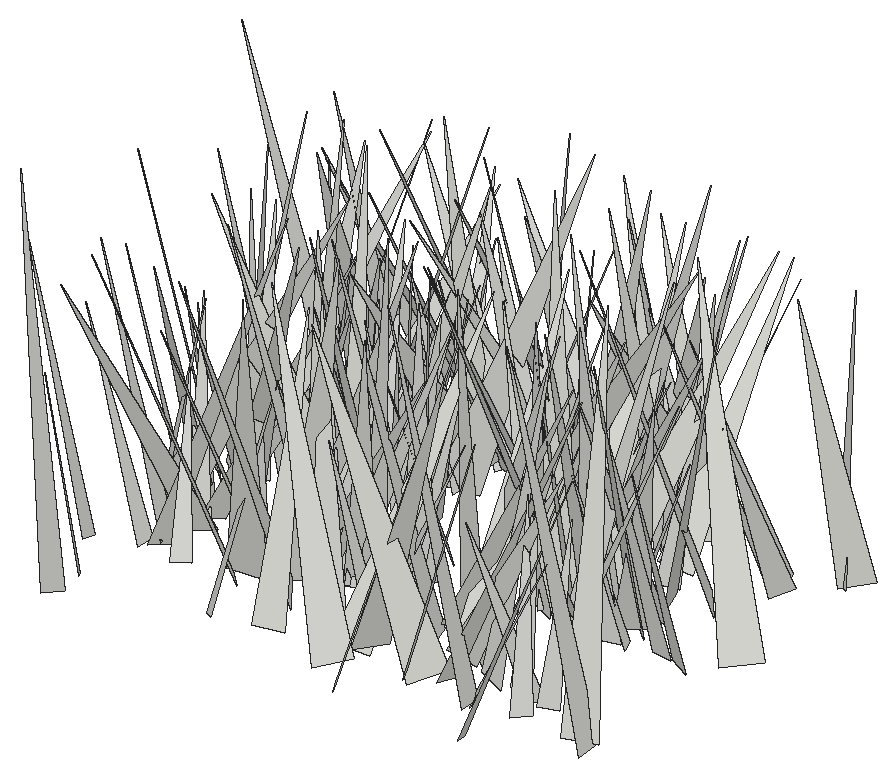
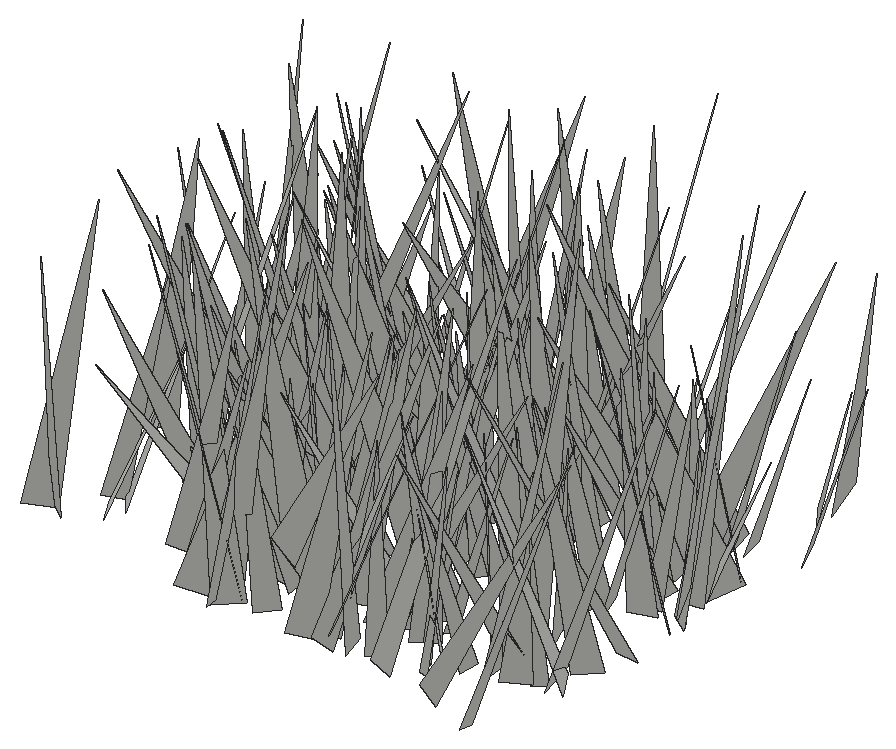
# SketchUp Ruby script. Lengths in inches.
U = 1.inch
M = Sketchup.active_model
def pt(a) = Geom::Point3d.new(a.map { |v| v * U })
def face(e, loops, mat)
  f = e.add_face(loops[0].map { |a| pt(a) })
  loops[1..].each { |l| e.add_face(l.map { |a| pt(a) }).erase! }
  f.material = f.back_material = mat if mat
  f
end
# faces: each face lists its corners as indices into pts; further lists are holes
def faces(e, pts, list, mat = nil) = list.each { |f| face(e, (f[0].is_a?(Array) ? f : [f]).map { |l| l.map { |i| pts[i] } }, mat) }
# xy, xz, yz: faces in a plane at the given z, y or x. An outline is a flat list of corners, or four numbers for a rectangle; further outlines are holes
def ring(l) = l.size == 4 ? [[l[0], l[1]], [l[2], l[1]], [l[2], l[3]], [l[0], l[3]]] : l.each_slice(2).to_a
def flat(e, list, mat, &to3) = list.each { |f| face(e, (f[0].is_a?(Array) ? f : [f]).map { |l| ring(l).map { |u, v| to3.(u, v) } }, mat) }
def xy(e, z, list, mat = nil) = flat(e, list, mat) { |x, y| [x, y, z] }
def xz(e, y, list, mat = nil) = flat(e, list, mat) { |x, z| [x, y, z] }
def yz(e, x, list, mat = nil) = flat(e, list, mat) { |y, z| [x, y, z] }
def lines(e, pts, list) = list.each { |a, b| e.add_line(pt(pts[a]), pt(pts[b])) }
# prism: a flat outline (further loops are holes) pulled along v
def prism(e, loops, v, mat = nil)
  f = face(e, loops, mat); d = Geom::Vector3d.new(v.map { |x| x * U })
  f.pushpull(f.normal.samedirection?(d) ? d.length : -d.length)
end
def box(e, o, s, mat = nil) = prism(e, [[o, [o[0] + s[0], o[1], o[2]], [o[0] + s[0], o[1] + s[1], o[2]], [o[0], o[1] + s[1], o[2]]]], [0, 0, s[2]], mat)
def at(x, y, z, deg = 0) = Geom::Transformation.translation(pt([x, y, z])) * Geom::Transformation.rotation(ORIGIN, Z_AXIS, deg.degrees)
def axes(o, x, y, z) = Geom::Transformation.new([*x, 0, *y, 0, *z, 0, *pt(o).to_a, 1])
def part(name) = M.definitions.add(name)
# library, detail: a bought-in or finely detailed component or shape, given as its bounding box
def library(name, o, s) = part(name).tap { |d| box(d.entities, o, s) }
def detail(e, o, s) = box(e.add_group.entities, o, s)
def put(e, d, t, mat = nil) = e.add_instance(d, t).tap { |i| i.material = mat if mat }
def group(e, t, mat = nil) = e.add_group.tap { |g| g.transformation = t; g.material = mat if mat }.entities
root = M.entities
c1 = part("fur_instance\#9")
p = [[0.8125,0,1.79],[0.67,-0.02,1.48],[0,-0.11,0],[0,0.11,0]]
faces(c1.entities,p,[[0,1,2,3]])
put(root,c1,axes([66.11,216.6875,-27.1],[-3.1769,-1.92196,0.83625],[-2.09296,2.82701,-1.45378],[-0.11299,1.67333,3.4166]))
put(root,c1,axes([66.16,215.04,-27.1],[-7.80069,-0.47128,0.71432],[-0.70737,7.23754,-2.94972],[0.48165,2.99651,7.23686]))
put(root,c1,axes([73.01,220.41,-27.1],[-6.10663,-5.12788,1.30944],[-4.81653,6.21333,1.86984],[2.19336,-0.63253,7.75176]))
put(root,c1,axes([80.8,218.62,-27.1],[-5.74656,4.30747,2.03787],[4.75581,5.38477,2.02895],[0.29923,-2.86007,6.88916]))
put(root,c1,axes([84.56,215.84,-27.1],[4.68389,2.5085,0.46697],[2.25732,-4.52881,1.68637],[-1.1896,1.28326,5.03861]))
put(root,c1,axes([83.1,218.38,-27.1],[3.88446,1.51086,0.00017],[1.46105,-3.75628,-1.06181],[0.38475,-0.98965,4.03042]))
put(root,c1,axes([77.45,217.25,-27.1],[-6.20404,3.776,0.73856],[3.82283,6.20814,0.37243],[0.43544,-0.70326,7.25325]))
put(root,c1,axes([77.75,219.07,-27.1],[6.355,-3.28716,0.66061],[-3.33311,-6.3472,0.48096],[-0.36352,0.73183,7.13864]))
put(root,c1,axes([70.61,220.09,-27.1],[-5.16383,-5.19186,0.43743],[-5.2089,5.15828,-0.26709],[0.11856,0.49863,7.31773]))
put(root,c1,axes([70.88,220.5,-27.1],[2.24537,-6.9608,0.71668],[-6.96969,-2.1575,0.8813],[0.62434,0.94895,7.26069]))
put(root,c1,axes([88.74,218.05,-27.1],[-7.60093,-1.69118,1.08047],[-1.85126,7.54274,-1.21718],[0.77483,1.43129,7.69108]))
put(root,c1,axes([85,219.61,-27.1],[0.84597,-3.78981,1.14812],[-3.67965,-1.18614,-1.20406],[-1.46323,0.79177,3.69169]))
put(root,c1,axes([79.92,218.47,-27.1],[4.69401,2.26049,0.88712],[2.32694,-4.7392,-0.23643],[-0.69438,-0.60059,5.20458]))
put(root,c1,axes([83.23,217.99,-27.1],[-7.26619,-2.16018,0.91047],[-2.32448,7.02333,-1.88745],[0.30351,2.07347,7.34176]))
put(root,c1,axes([78.58,215.9375,-27.1],[6.47169,4.71895,0.84374],[4.29058,-6.33416,2.51645],[-2.13805,1.57262,7.60387]))
put(root,c1,axes([71.67,217.26,-27.1],[2.88186,3.44939,0.31018],[3.15851,-2.7832,1.60537],[-1.42067,0.8094,4.19835]))
put(root,c1,axes([85.27,218.45,-27.1],[-3.68366,1.92684,0.76086],[1.83141,3.75443,-0.64122],[0.96827,0.22919,4.10742]))
put(root,c1,axes([74.02,217.77,-27.1],[-1.14776,6.0133,0.84328],[6.0716,1.14805,0.07727],[0.08148,-0.84289,6.12137]))
put(root,c1,axes([67.57,222.01,-27.1],[0.6668,-6.36542,0.43774],[-6.10772,-0.7641,-1.80742],[-1.84553,0.22889,6.13974]))
put(root,c1,axes([85.68,219.51,-27.1],[-1.6026,3.32948,1.45838],[3.48573,1.8596,-0.41502],[1.03054,-1.11225,3.67172]))
put(root,c1,axes([80.87,220.48,-27.1],[2.62599,-5.06265,0.78885],[-4.77605,-2.09765,2.43674],[1.85526,1.76578,5.15641]))
put(root,c1,axes([76.58,220.64,-27.1],[-3.79793,-0.43925,1.06155],[-0.29859,3.91782,0.55288],[1.10936,-0.44932,3.78306]))
put(root,c1,axes([64.625,219.06,-27.1],[-5.41168,-1.42657,0.35166],[-1.45652,5.03228,-1.99993],[-0.1932,2.0214,5.22701]))
put(root,c1,axes([66.51,220.01,-27.1],[-4.63616,-0.58897,0.33378],[-0.62989,4.59941,-0.63319],[0.24806,0.67142,4.63033]))
put(root,c1,axes([83.89,220.2,-27.1],[-2.42915,2.39744,1.43013],[2.49267,2.71628,-0.31959],[1.25681,-0.75355,3.39799]))
put(root,c1,axes([81.48,218.91,-27.1],[6.28882,0.29269,0.74734],[0.08478,-6.11246,1.68051],[-0.79813,1.65699,6.06719]))
put(root,c1,axes([72.62,221.29,-27.1],[5.72788,-5.11466,1.67521],[-5.30647,-5.77538,0.51083],[-0.89854,1.50329,7.66207]))
put(root,c1,axes([74.9375,220.11,-27.1],[1.5886,-5.12639,3.23902],[-5.9044,-2.07062,-0.3813],[-1.38174,2.95423,5.35333]))
put(root,c1,axes([68.4375,219.66,-27.1],[-2.65941,2.49787,0.36396],[2.46932,2.68404,-0.37765],[0.52369,0.0288,3.62894]))
put(root,c1,axes([82.79,219.81,-27.1],[2.70818,5.99392,1.73773],[6.22026,-2.74585,-0.22279],[-0.5051,-1.67756,6.57356]))
put(root,c1,axes([88.07,218.36,-27.1],[-0.32528,8.12923,0.88129],[8.06717,0.17507,1.36272],[-1.33486,-0.92294,8.0208]))
put(root,c1,axes([69.37,222.66,-27.1],[-3.58338,-3.97137,0.418],[-3.89573,3.60001,0.80641],[0.87736,-0.23507,5.28792]))
put(root,c1,axes([74.7,222.36,-27.1],[2.07468,-5.92746,1.15005],[-6.03286,-1.98482,0.6533],[0.24901,1.299,6.24598]))
put(root,c1,axes([76.66,221.06,-27.1],[3.8277,2.64651,0.3376],[2.6435,-3.68235,-1.10521],[0.36045,-1.09797,4.52038]))
put(root,c1,axes([66.93,220.8,-27.1],[-5.59376,-1.56322,0.76508],[-1.67452,5.53596,-0.93185],[0.47433,1.10847,5.73284]))
put(root,c1,axes([79.26,221.17,-27.1],[-7.24522,-3.15461,1.03201],[-3.28219,7.17812,-1.10079],[0.49381,1.42581,7.82516]))
put(root,c1,axes([73.9375,221.45,-27.1],[-6.93543,-2.32629,0.88421],[-2.41004,6.93097,-0.66862],[0.62063,0.91853,7.28456]))
put(root,c1,axes([75.76,221.72,-27.1],[-2.07525,-6.86081,3.30693],[-7.48887,2.46229,0.40886],[1.38687,3.02978,7.15613]))
put(root,c1,axes([72.81,222.07,-27.1],[4.53332,-3.78068,0.06575],[-3.6354,-4.32956,1.69931],[1.04008,1.34544,5.65304]))
put(root,c1,axes([65.54,224.64,-27.1],[-1.80775,-6.68688,0.47497],[-6.40102,1.86794,1.93536],[1.9917,-0.06601,6.65106]))
put(root,c1,axes([77.28,218.5,-27.1],[-4.67484,5.38464,0.57126],[4.73589,4.43174,-3.01759],[2.62527,1.59378,6.46085]))
put(root,c1,axes([65.61,221.8,-27.1],[3.51843,3.11531,1.14482],[3.25687,-3.56198,-0.31656],[-0.63919,-1.00114,4.68874]))
put(root,c1,axes([84.57,222.4,-27.1],[-3.5972,0.42819,0.55364],[0.48536,3.61469,0.35791],[0.50428,-0.42464,3.60487]))
put(root,c1,axes([67.03,220.26,-27.1],[6.5419,0.41912,1.71437],[-0.23349,-6.31856,2.43568],[-1.74935,2.41069,6.08602]))
put(root,c1,axes([72.625,222.8,-27.1],[-4.98307,4.13485,3.06586],[4.6284,5.46651,0.15019],[2.25263,-2.08511,6.47344]))
put(root,c1,axes([83.41,224.29,-27.1],[-4.28269,-7.03673,0.88853],[-7.06243,4.13524,-1.29164],[-0.65353,1.42504,8.13564]))
put(root,c1,axes([73.49,221.21,-27.1],[1.79121,4.66243,0.42191],[4.67903,-1.79759,0.00003],[-0.15134,-0.39383,4.99466]))
put(root,c1,axes([73.9375,222.66,-27.1],[3.63408,5.21962,1.38175],[5.32326,-3.18476,-1.96987],[0.90365,-2.23003,6.04736]))
put(root,c1,axes([73.88,224.8,-27.1],[-3.21608,-6.87634,1.40534],[-6.91778,3.36666,0.64196],[1.18463,0.99184,7.56406]))
put(root,c1,axes([69.6,221.78,-27.1],[-4.54245,-0.30979,1.16713],[-0.64985,4.4561,-1.34644],[1.01777,1.46262,4.34936]))
put(root,c1,axes([67.3,224.73,-27.1],[7.07591,-3.11018,0.05148],[-3.09924,-7.06002,-0.5432],[-0.26559,-0.47663,7.71016]))
put(root,c1,axes([67.09,222.4,-27.1],[-1.17354,4.22506,1.16991],[4.38332,1.15287,0.2334],[0.0799,-1.19029,4.3788]))
put(root,c1,axes([79.09,222.35,-27.1],[5.6454,-1.61471,0.55375],[-1.70236,-5.46688,1.41409],[-0.12614,1.5134,5.69896]))
put(root,c1,axes([78.53,224.375,-27.1],[5.01746,5.30698,2.27397],[5.71554,-4.13917,-2.95123],[0.81705,-3.63499,6.68051]))
put(root,c1,axes([76.23,223.79,-27.1],[4.61817,-3.87726,2.02523],[-4.05143,-4.90172,-0.14567],[-1.64942,1.18414,6.02822]))
put(root,c1,axes([84.08,226.64,-27.1],[-3.7888,-7.35051,1.42507],[-6.56657,4.02946,3.32556],[3.59735,-0.38635,7.57137]))
put(root,c1,axes([81.83,220.48,-27.1],[4.6203,4.92142,0.32663],[4.69042,-4.52255,1.79463],[-1.52544,1.00021,6.50745]))
put(root,c1,axes([83.48,223.43,-27.1],[5.31801,3.62577,0.57345],[3.65614,-5.14142,-1.39812],[0.32822,-1.47507,6.28273]))
put(root,c1,axes([65.12,225.94,-27.1],[-4.90749,-6.3294,1.61985],[-6.13533,5.16095,1.5783],[2.24565,0.26836,7.85199]))
put(root,c1,axes([87.46,224.91,-27.1],[-1.94034,-4.30134,0.80925],[-4.30819,2.03312,0.47669],[0.77193,0.53502,4.69459]))
put(root,c1,axes([71.875,222.58,-27.1],[6.69974,-1.69034,1.74311],[-2.11177,-6.58131,1.73465],[-1.19837,2.1474,6.68841]))
put(root,c1,axes([80.61,225.22,-27.1],[-1.45623,-6.82166,1.9418],[-6.84757,1.86878,1.42991],[1.84835,1.54881,6.82723]))
put(root,c1,axes([70.27,221.8,-27.1],[-6.71472,0.14595,1.05093],[-0.21339,6.41005,-2.25365],[1.03933,2.25902,6.32691]))
put(root,c1,axes([72.54,224.67,-27.1],[-7.38136,0.22251,0.33251],[0.26326,7.32737,0.9407],[0.30128,-0.95116,7.32455]))
put(root,c1,axes([66.55,225.73,-27.1],[-0.44013,-4.40012,0.04518],[-4.35564,0.44209,0.62427],[0.62566,-0.01764,4.37779]))
put(root,c1,axes([78.22,224.39,-27.1],[-1.72933,-6.01967,2.37326],[-6.41752,1.90965,0.16749],[0.82719,2.23073,6.26091]))
put(root,c1,axes([65.21,223.27,-27.1],[6.5519,-4.81181,0.9912],[-4.80718,-5.93833,2.94799],[1.01342,2.94042,7.57563]))
put(root,c1,axes([82.35,225.16,-27.1],[4.90048,2.76624,3.25214],[3.64641,-5.28694,-0.99757],[-2.22086,-2.5767,5.5382]))
put(root,c1,axes([74.45,222.36,-27.1],[-5.1152,1.11044,1.16629],[0.73583,5.06638,-1.59654],[1.43244,1.36283,4.98492]))
put(root,c1,axes([76.2,223.375,-27.1],[1.29664,4.3065,0.97913],[4.41517,-1.23995,-0.39328],[0.1042,-1.05001,4.48024]))
put(root,c1,axes([75.55,224.12,-27.1],[-4.97388,0.03891,0.99351],[0.0174,5.07103,-0.11152],[0.99411,0.10595,4.97278]))
put(root,c1,axes([75.82,226.16,-27.1],[-3.10311,-4.08719,0.56583],[-3.96021,3.14894,1.02739],[1.15846,-0.18348,5.02781]))
put(root,c1,axes([86.49,225.13,-27.1],[-1.41742,-4.71426,1.18858],[-4.85717,1.31918,-0.56008],[-0.21176,1.29675,4.89077]))
put(root,c1,axes([80.7,223.43,-27.1],[3.10796,2.24348,0.34109],[2.21254,-3.12436,0.38987],[-0.50422,0.11876,3.81322]))
put(root,c1,axes([82.67,225.86,-27.1],[-2.15861,-6.19615,1.53511],[-6.31129,2.3146,0.46773],[0.95736,1.28794,6.5447]))
put(root,c1,axes([65.81,223.35,-27.1],[-4.45593,-2.02584,0.38216],[-1.95722,3.87117,-2.29973],[-0.64758,2.23951,4.32095]))
put(root,c1,axes([71.12,227.32,-27.1],[-1.84691,-6.18778,0.26193],[-5.9057,1.84189,1.87043],[1.86547,-0.29517,6.18071]))
put(root,c1,axes([80.29,222.14,-27.1],[-2.04424,6.85145,0.72305],[6.79433,2.1298,-0.97223],[1.1412,-0.40704,7.08351]))
put(root,c1,axes([84.32,226.03,-27.1],[4.15858,-4.6502,0.45845],[-4.67236,-4.14601,0.32855],[-0.05962,0.56087,6.22978]))
put(root,c1,axes([85.04,224.92,-27.1],[-3.24657,-1.58505,0.39086],[-1.61743,3.24104,-0.29141],[0.22149,0.43432,3.60107]))
put(root,c1,axes([66.27,224.1,-27.1],[1.10778,3.32388,1.25845],[3.28018,-1.46364,0.97838],[-1.36832,-0.8177,3.36424]))
put(root,c1,axes([74.29,222.03,-27.1],[0.27633,8.1596,0.76138],[7.93766,-0.45592,2.00518],[-2.0377,-0.66947,7.91421]))
put(root,c1,axes([67.32,222.95,-27.1],[6.04009,-0.71684,0.90558],[-1.00409,-5.64184,2.23115],[-0.57074,2.3393,5.65849]))
put(root,c1,axes([75.07,224.62,-27.1],[3.97041,-1.42005,1.05601],[-1.57618,-4.01704,0.5243],[-0.80459,0.86179,4.18399]))
put(root,c1,axes([82.32,226.71,-27.1],[3.11086,-6.46121,1.0779],[-6.53922,-3.13316,0.09147],[-0.38422,1.01124,7.17051]))
put(root,c1,axes([84.72,227.09,-27.1],[-0.49515,-5.81147,0.35136],[-5.82208,0.49376,-0.03799],[-0.0081,0.35331,5.8324]))
put(root,c1,axes([84.35,224.77,-27.1],[-0.90978,-4.59674,2.27002],[-5.08569,0.51819,-0.98893],[-0.64715,2.39002,4.58036]))
put(root,c1,axes([66.72,224.68,-27.1],[3.29977,-2.51906,0.3221],[-2.3698,-2.86445,1.87534],[0.91296,1.66948,3.70368]))
put(root,c1,axes([65.06,225.91,-27.1],[-2.14945,-3.42966,1.0737],[-3.50191,2.27993,0.27214],[0.80747,0.75821,4.03839]))
put(root,c1,axes([73.53,223.98,-27.1],[-4.06355,5.05875,1.67662],[5.05755,4.32523,-0.79246],[1.68023,-0.78477,6.44014]))
put(root,c1,axes([83.28,223.7,-27.1],[2.96798,6.81466,1.03357],[6.887,-2.97737,-0.1458],[-0.27767,-1.00619,7.4315]))
put(root,c1,axes([71.31,223.18,-27.1],[2.8075,7.47142,1.47372],[7.21104,-3.11318,2.04573],[-2.44844,-0.60171,7.71486]))
put(root,c1,axes([67.65,224.5,-27.1],[-6.13991,-1.94187,2.86824],[-2.65031,6.39227,-1.34568],[2.23013,2.25037,6.2975]))
put(root,c1,axes([68.13,226.78,-27.1],[4.67852,-1.7119,0.20248],[-1.71617,-4.68064,0.08066],[-0.16239,0.14538,4.98123]))
put(root,c1,axes([80.99,227.23,-27.1],[-3.56669,-5.90918,0.59479],[-5.71236,3.22345,-2.22975],[-1.62517,1.63841,6.53207]))
put(root,c1,axes([74.39,226.35,-27.1],[4.38059,2.58911,2.20412],[2.75267,-4.81057,0.18002],[-1.99611,-0.9519,5.08534]))
put(root,c1,axes([81.25,225.6875,-27.1],[-7.16118,3.19135,1.99245],[3.1192,7.43157,-0.69239],[2.1036,-0.15533,7.80947]))
put(root,c1,axes([66.59,226.27,-27.1],[-1.35199,5.16754,1.66066],[5.39955,1.4549,-0.13134],[0.55327,-1.57128,5.33986]))
put(root,c1,axes([73.99,227.46,-27.1],[5.32416,0.8497,1.29821],[1.01973,-5.41351,-0.63884],[-1.1694,-0.85204,5.35356]))
put(root,c1,axes([70.57,228.54,-27.1],[4.90607,-3.46037,0.24315],[-3.44997,-4.91123,-0.28332],[-0.36191,-0.09172,5.99695]))
put(root,c1,axes([72.83,227.625,-27.1],[2.7967,-3.72992,1.22325],[-3.91864,-2.74089,0.60164],[-0.23004,1.34365,4.62297]))
put(root,c1,axes([85.49,229.33,-27.1],[-6.16047,-5.25921,0.96963],[-5.25018,6.22911,0.42963],[1.01736,0.29959,8.08864]))
put(root,c1,axes([67.79,226.75,-27.1],[-6.22819,-1.34042,0.61243],[-1.44458,6.07908,-1.38568],[0.29149,1.48668,6.21828]))
put(root,c1,axes([77.65,230.31,-27.1],[-1.30326,-6.4856,0.41929],[-6.05179,1.36694,2.33336],[2.36951,-0.07596,6.19006]))
put(root,c1,axes([72.81,231.78,-27.1],[6.08431,-4.17162,0.61258],[-3.3903,-5.47976,-3.64343],[-2.50671,-2.71408,6.41457]))
put(root,c1,axes([89.14,226.45,-27.1],[-5.24663,5.623,0.95369],[5.70188,5.20042,0.70642],[0.12741,-1.17997,7.65808]))
put(root,c1,axes([65.54,226.18,-27.1],[4.64173,5.41011,1.53464],[5.42173,-4.8336,0.64123],[-1.49305,-0.73288,7.09956]))
put(root,c1,axes([82.8,228.55,-27.1],[3.70621,1.73352,0.50221],[1.78343,-3.34171,-1.62653],[0.27688,-1.67963,3.75439]))
put(root,c1,axes([69.34,226.6,-27.1],[-4.14484,-0.82966,2.07391],[-1.4546,4.32013,-1.17886],[1.69516,1.67847,4.05935]))
put(root,c1,axes([84.28,228.34,-27.1],[6.26752,1.77798,1.53658],[2.00319,-6.33057,-0.84565],[-1.22862,-1.25168,6.45971]))
put(root,c1,axes([77.41,228.84,-27.1],[3.81653,-4.78014,0.36891],[-4.62204,-3.54318,1.90641],[1.2738,1.46558,5.81217]))
put(root,c1,axes([78.375,227.81,-27.1],[-1.43576,4.62376,1.24523],[4.74317,1.1948,1.0324],[-0.65727,-1.47798,4.73019]))
put(root,c1,axes([80.45,228.65,-27.1],[5.56558,-2.4926,0.3103],[-2.49513,-5.39934,1.38077],[0.28926,1.38533,5.93988]))
put(root,c1,axes([77.3,230.41,-27.1],[-3.93498,0.71077,2.15609],[1.47172,4.08376,1.33974],[1.72857,-1.85895,3.76754]))
put(root,c1,axes([76.67,229.36,-27.1],[6.17977,-5.38552,0.13557],[-5.06059,-5.73249,2.95646],[1.84733,2.31224,7.64543]))
put(root,c1,axes([71.3,228.38,-27.1],[2.20928,6.37096,1.50715],[6.50914,-1.9672,-1.22586],[0.70121,-1.81177,6.63078]))
put(root,c1,axes([78.35,230.31,-27.1],[0.55845,-3.67703,0.59896],[-3.72525,-0.55803,0.04757],[-0.0423,0.59936,3.71889]))
put(root,c1,axes([83.42,229.3125,-27.1],[-1.45732,3.49071,1.72371],[3.67662,1.83923,-0.61623],[1.28012,-1.30851,3.73217]))
put(root,c1,axes([82.125,227.47,-27.1],[-6.70082,0.16595,0.10129],[0.12128,6.29761,-2.29436],[0.15195,2.29157,6.29797]))
put(root,c1,axes([66.8125,233.06,-27.1],[7.11754,-4.23376,0.53848],[-3.90576,-6.88369,-2.49681],[-1.7204,-1.88792,7.89621]))
put(root,c1,axes([81.8,227.51,-27.1],[-0.75445,7.6495,1.46212],[7.18414,1.25072,-2.83648],[3.00677,-1.06897,7.14412]))
put(root,c1,axes([73.04,230.39,-27.1],[-4.43499,0.78648,1.49873],[1.10021,4.53377,0.87655],[1.28619,-1.16631,4.41807]))
put(root,c1,axes([80.39,228.39,-27.1],[-1.23415,4.06964,0.18802],[4.01431,1.18128,0.78126],[-0.69473,-0.40381,4.18028]))
put(root,c1,axes([87,231.48,-27.1],[3.36953,-3.09183,0.80409],[-2.80421,-3.42236,-1.4084],[-1.53048,-0.53643,4.35081]))
put(root,c1,axes([70.37,227.78,-27.1],[6.70956,3.50603,1.11128],[3.28027,-6.75003,1.49074],[-1.66343,0.8308,7.42214]))
put(root,c1,axes([86.29,231.69,-27.1],[-4.87517,-3.87645,0.62854],[-3.83008,4.91477,0.6039],[0.86741,-0.08574,6.19915]))
put(root,c1,axes([68.71,231.24,-27.1],[3.22144,-2.0672,0.86258],[-1.86043,-3.31076,-0.98626],[-1.24746,-0.40075,3.69841]))
put(root,c1,axes([80.44,229.1875,-27.1],[3.75823,0.40452,0.85087],[0.18545,-3.74836,0.96295],[-0.9237,0.89332,3.65522]))
put(root,c1,axes([80.23,229.37,-27.1],[-3.57041,1.71359,0.7726],[1.61509,3.64514,-0.62093],[0.96166,0.24019,3.91135]))
put(root,c1,axes([71.13,231.71,-27.1],[-3.68775,-0.43694,1.2324],[0.03671,3.65173,1.40455],[1.30705,-1.33536,3.43768]))
put(root,c1,axes([78.8125,230.26,-27.1],[3.29309,2.39527,0.08068],[2.3726,-3.23886,-0.68467],[0.3385,-0.60058,4.0141]))
put(root,c1,axes([67.92,229.49,-27.1],[-5.24858,-0.93793,1.2858],[-1.33069,5.01688,-1.77222],[0.87308,2.00792,5.02857]))
put(root,c1,axes([72.91,230.14,-27.1],[5.54256,-5.39998,2.31392],[-5.86744,-4.92827,2.55329],[0.29519,3.43313,7.30483]))
put(root,c1,axes([76.33,231.03,-27.1],[-4.97411,1.9133,1.24146],[2.05101,5.05519,0.42681],[0.99764,-0.85328,5.31228]))
put(root,c1,axes([74.58,234.39,-27.1],[-5.86145,-3.99032,0.23805],[-3.68658,5.55942,2.41617],[1.54546,-1.87245,6.66644]))
put(root,c1,axes([75.2,232.19,-27.1],[3.86572,-4.28586,2.24353],[-4.19582,-4.39988,-1.17556],[-2.40771,0.7863,5.6507]))
put(root,c1,axes([81.4,231.87,-27.1],[-6.84332,-0.22544,2.15666],[-0.013,7.14388,0.70553],[2.16837,-0.66867,6.81058]))
put(root,c1,axes([65.02,229.11,-27.1],[2.4491,6.4359,0.09226],[6.32974,-2.3903,-1.28384],[1.16776,-0.54137,6.7654]))
put(root,c1,axes([78.89,229.03,-27.1],[-1.68385,4.77561,0.18208],[4.53538,1.65768,-1.53538],[1.50664,0.34725,4.82539]))
put(root,c1,axes([69.54,231.35,-27.1],[3.09242,2.58599,1.68004],[2.84079,-3.31463,-0.12697],[-1.19992,-1.18273,4.02918]))
put(root,c1,axes([66.19,232.72,-27.1],[-0.42992,-4.68733,0.89248],[-4.33891,0.75688,1.88505],[1.98531,0.63912,4.31306]))
put(root,c1,axes([82.04,231.91,-27.1],[4.94298,-3.20176,1.42299],[-3.34359,-5.04595,0.26096],[-1.0472,0.99819,5.88356]))
put(root,c1,axes([73.31,232.36,-27.1],[-3.41079,-4.86692,0.40111],[-4.72199,3.16213,-1.78467],[-1.24525,1.33989,5.66881]))
put(root,c1,axes([81.04,228.74,-27.1],[-5.5806,3.5391,0.90465],[3.04631,5.42049,-2.4135],[2.01583,1.60617,6.15169]))
put(root,c1,axes([65.36,230.97,-27.1],[2.82826,-4.43632,2.67471],[-5.15951,-2.68482,1.00262],[-0.46309,2.81866,5.16476]))
put(root,c1,axes([86.58,232.45,-27.1],[-4.47388,-2.50611,0.21033],[-2.51468,4.46372,-0.30343],[0.03476,0.36756,5.119]))
put(root,c1,axes([76.38,232.27,-27.1],[-4.16703,-2.76107,2.92288],[-2.78486,5.0182,0.77013],[2.90022,0.85149,4.93909]))
put(root,c1,axes([80.46,235.11,-27.1],[3.62515,-5.36286,0.15908],[-5.03579,-3.46731,-2.13211],[-1.85105,-1.06996,6.11196]))
put(root,c1,axes([77.58,232.02,-27.1],[6.54433,-2.87567,1.841],[-3.10892,-6.66403,0.64215],[-1.41189,1.3447,7.11937]))
put(root,c1,axes([81.07,231.58,-27.1],[3.79421,5.57197,1.64798],[5.81056,-3.63804,-1.07735],[0.00109,-1.96889,6.65448]))
put(root,c1,axes([71.54,235.33,-27.1],[-3.81436,-7.20009,0.2192],[-7.12697,3.80817,1.069],[1.0467,-0.30859,8.07762]))
put(root,c1,axes([72.45,232.22,-27.1],[-6.37075,2.32719,2.17346],[2.54476,6.64308,0.34616],[1.91413,-1.08621,6.77365]))
put(root,c1,axes([79.44,230.89,-27.1],[7.05742,-1.09775,2.22467],[-1.64487,-7.09246,1.71837],[-1.85705,2.1103,6.93249]))
put(root,c1,axes([75.16,229.98,-27.1],[4.59925,2.87418,0.36346],[2.61006,-4.40682,1.82035],[-1.25721,1.36572,5.10885]))
put(root,c1,axes([68.05,233.23,-27.1],[-6.59248,-1.12335,1.64682],[-1.04061,6.79216,0.46743],[1.70031,-0.1986,6.67115]))
put(root,c1,axes([66,232,-27.1],[-7.51977,-1.08655,0.44758],[-1.14316,7.43533,-1.15625],[0.27218,1.20961,7.50937]))
put(root,c1,axes([73.45,232.79,-27.1],[-4.72001,4.32069,1.36462],[4.52973,4.45158,1.57294],[-0.11027,-2.07946,6.20264]))
put(root,c1,axes([88.76,233.65,-27.1],[3.4747,-4.84053,2.29693],[-4.84614,-4.00697,-1.11322],[-2.28507,1.13736,5.85363]))
put(root,c1,axes([71.45,232.82,-27.1],[2.88206,-3.90926,2.29022],[-4.22914,-3.29495,-0.30223],[-1.62535,1.64154,4.8474]))
put(root,c1,axes([74.39,235.25,-27.1],[-1.51656,-6.50321,0.08888],[-6.50028,1.51258,-0.24097],[-0.21452,0.14123,6.67335]))
put(root,c1,axes([77.62,232.66,-27.1],[3.69637,0.13401,0.11411],[0.12786,-3.69317,0.19555],[-0.12096,0.19138,3.69362]))
put(root,c1,axes([82.78,230.53,-27.1],[-1.93845,6.02083,0.54238],[5.77969,2.01278,-1.68701],[1.77192,0.02133,6.09606]))
put(root,c1,axes([80.57,232.4,-27.1],[4.17066,5.06918,1.33611],[5.23853,-4.09478,-0.81653],[-0.19883,-1.55319,6.51339]))
put(root,c1,axes([71.9375,231.21,-27.1],[-3.2921,4.67046,0.35788],[4.62081,3.30978,-0.68745],[0.76768,0.10645,5.67261]))
put(root,c1,axes([78.93,232.55,-27.1],[-3.29072,5.65648,0.59206],[5.32719,2.82602,2.60955],[-1.99181,-1.7869,6.00123]))
put(root,c1,axes([78.8125,235.04,-27.1],[1.7793,-6.50243,0.4842],[-6.28195,-1.575,1.93351],[1.74732,0.95904,6.45825]))
put(root,c1,axes([70.05,234.69,-27.1],[-2.01295,-3.23513,0.63988],[-3.06607,2.112,1.03257],[1.21439,-0.03018,3.66768]))
put(root,c1,axes([77.38,234.61,-27.1],[2.01974,-4.62687,0.27657],[-4.52399,-1.90214,1.21619],[1.00891,0.73329,4.89981]))
put(root,c1,axes([69.64,233.98,-27.1],[4.05743,2.55482,1.17911],[2.80714,-3.81746,-1.3882],[-0.19333,-1.81108,4.58942]))
put(root,c1,axes([81.21,234.22,-27.1],[3.41803,-2.18502,2.15563],[-1.95303,-4.03718,-0.99543],[-2.36786,0.1758,3.93273]))
put(root,c1,axes([72.18,234.72,-27.1],[1.68223,-3.64936,0.16027],[-3.63941,-1.65928,0.41825],[0.31341,0.31999,3.9966]))
put(root,c1,axes([75.18,235.29,-27.1],[2.93992,-5.13493,1.13143],[-5.01799,-3.12719,-1.15379],[-1.5708,0.37938,5.8034]))
put(root,c1,axes([82.6,232.98,-27.1],[-2.33709,5.71521,1.48586],[5.84354,2.00796,1.46781],[-0.85111,-1.90732,5.99759]))
put(root,c1,axes([68.98,233.375,-27.1],[3.85375,-0.57416,0.66525],[-0.65849,-3.86826,0.47595],[-0.58191,0.57487,3.8671]))
put(root,c1,axes([74.52,234.52,-27.1],[0.87067,-3.63818,0.96208],[-3.64876,-1.05785,-0.69825],[-0.92116,0.75142,3.67517]))
put(root,c1,axes([65.48,232.125,-27.1],[5.06961,3.19969,0.78256],[3.08145,-5.11429,0.94868],[-1.16407,0.39664,5.91937]))
put(root,c1,axes([78.72,234.52,-27.1],[3.57739,2.98141,0.96801],[3.07785,-3.06266,-1.94177],[0.59384,-2.08684,4.23274]))
put(root,c1,axes([79.36,235.24,-27.1],[-5.69321,-2.11736,2.09192],[-1.78965,6.04293,1.24584],[2.37833,-0.52131,5.94506]))
put(root,c1,axes([82.03,230.68,-27.1],[4.84887,3.21318,0.05137],[2.84684,-4.33809,2.62966],[-1.49084,2.16682,5.18854]))
put(root,c1,axes([67.26,232.38,-27.1],[0.04423,5.29855,0.55334],[5.02486,0.14232,-1.76445],[1.76963,-0.53655,4.99632]))
put(root,c1,axes([75.43,233.31,-27.1],[-5.24793,-3.08562,0.82091],[-3.15493,4.76816,-2.24651],[-0.49124,2.34081,5.65818]))
put(root,c1,axes([88.2,233.4,-27.1],[2.88835,4.68484,1.93004],[4.79823,-3.24275,0.69058],[-1.62782,-1.24585,5.46016]))
put(root,c1,axes([80.03,233.75,-27.1],[-2.9661,5.6248,1.68099],[5.86235,2.73802,1.18234],[-0.31135,-2.03143,6.24805]))
put(root,c1,axes([68.92,235.83,-27.1],[-2.19806,-5.17129,0.07017],[-4.98418,2.09779,-1.52836],[-1.38027,0.66005,5.4072]))
put(root,c1,axes([70.94,233.36,-27.1],[2.36274,4.29484,1.97791],[3.91667,-3.01643,1.87116],[-2.64906,-0.62918,4.53067]))
put(root,c1,axes([73.29,234.74,-27.1],[6.28919,2.00514,2.27548],[2.25266,-6.59596,-0.4138],[-2.03074,-1.10685,6.58812]))
put(root,c1,axes([66.37,236.8,-27.1],[-5.34659,-1.99732,0.9572],[-1.60106,5.21354,1.93576],[1.5304,-1.52357,5.36919]))
